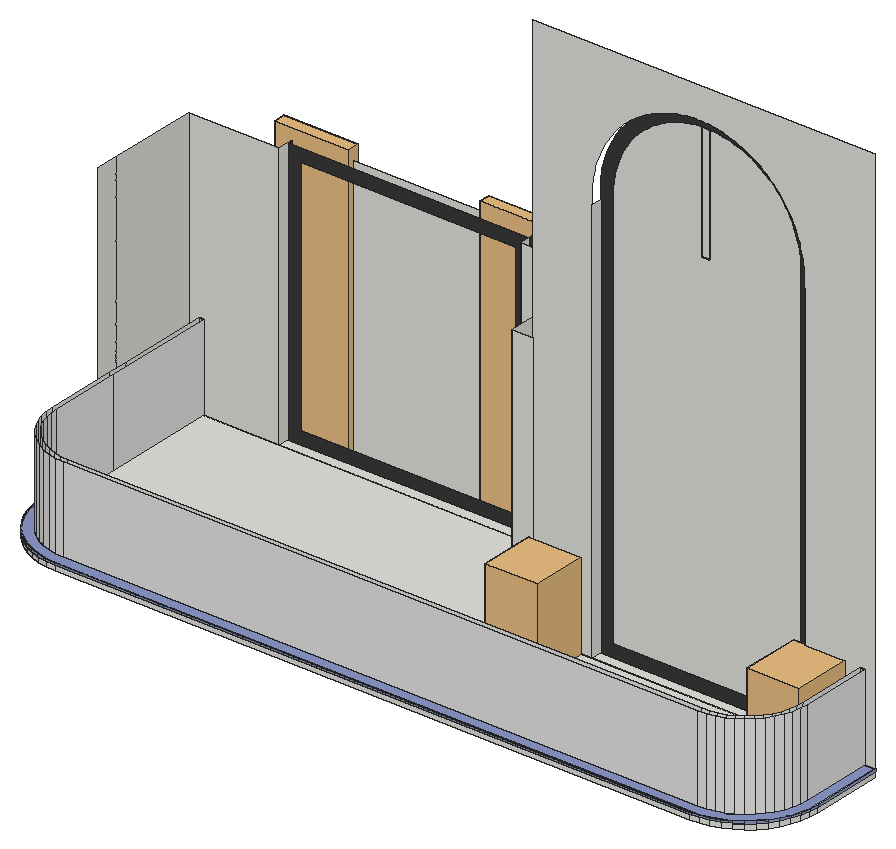
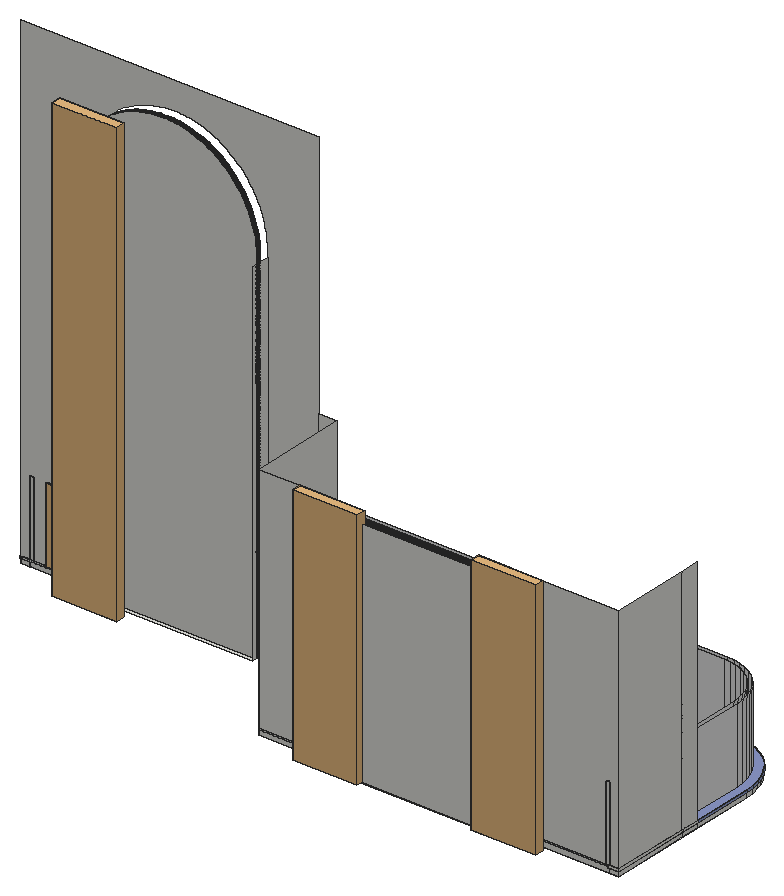
# SketchUp Ruby script. Lengths in inches.
U = 1.inch
M = Sketchup.active_model
def pt(a) = Geom::Point3d.new(a.map { |v| v * U })
def face(e, loops, mat)
  f = e.add_face(loops[0].map { |a| pt(a) })
  loops[1..].each { |l| e.add_face(l.map { |a| pt(a) }).erase! }
  f.material = f.back_material = mat if mat
  f
end
# faces: each face lists its corners as indices into pts; further lists are holes
def faces(e, pts, list, mat = nil) = list.each { |f| face(e, (f[0].is_a?(Array) ? f : [f]).map { |l| l.map { |i| pts[i] } }, mat) }
# xy, xz, yz: faces in a plane at the given z, y or x. An outline is a flat list of corners, or four numbers for a rectangle; further outlines are holes
def ring(l) = l.size == 4 ? [[l[0], l[1]], [l[2], l[1]], [l[2], l[3]], [l[0], l[3]]] : l.each_slice(2).to_a
def flat(e, list, mat, &to3) = list.each { |f| face(e, (f[0].is_a?(Array) ? f : [f]).map { |l| ring(l).map { |u, v| to3.(u, v) } }, mat) }
def xy(e, z, list, mat = nil) = flat(e, list, mat) { |x, y| [x, y, z] }
def xz(e, y, list, mat = nil) = flat(e, list, mat) { |x, z| [x, y, z] }
def yz(e, x, list, mat = nil) = flat(e, list, mat) { |y, z| [x, y, z] }
def lines(e, pts, list) = list.each { |a, b| e.add_line(pt(pts[a]), pt(pts[b])) }
# prism: a flat outline (further loops are holes) pulled along v
def prism(e, loops, v, mat = nil)
  f = face(e, loops, mat); d = Geom::Vector3d.new(v.map { |x| x * U })
  f.pushpull(f.normal.samedirection?(d) ? d.length : -d.length)
end
def box(e, o, s, mat = nil) = prism(e, [[o, [o[0] + s[0], o[1], o[2]], [o[0] + s[0], o[1] + s[1], o[2]], [o[0], o[1] + s[1], o[2]]]], [0, 0, s[2]], mat)
def at(x, y, z, deg = 0) = Geom::Transformation.translation(pt([x, y, z])) * Geom::Transformation.rotation(ORIGIN, Z_AXIS, deg.degrees)
def axes(o, x, y, z) = Geom::Transformation.new([*x, 0, *y, 0, *z, 0, *pt(o).to_a, 1])
def part(name) = M.definitions.add(name)
# library, detail: a bought-in or finely detailed component or shape, given as its bounding box
def library(name, o, s) = part(name).tap { |d| box(d.entities, o, s) }
def detail(e, o, s) = box(e.add_group.entities, o, s)
def put(e, d, t, mat = nil) = e.add_instance(d, t).tap { |i| i.material = mat if mat }
def group(e, t, mat = nil) = e.add_group.tap { |g| g.transformation = t; g.material = mat if mat }.entities
root = M.entities
M.materials.add("0326 AP 7207 CLASSIC PURPLE").color = [140, 152, 201]
M.materials.add("[Color M07]").color = [58, 58, 58]
M.materials.add("[Mirror 02]").color = [229, 229, 229]
c1 = library("Curtains 004",[-15.59,-2.26,0],[31.18,4.52,116.91])
c2 = library("Ficus elastica Belize 002",[-7.92,-8.8125,0.01],[22.14,24.73,36.43])
xy(root,136.75,[[220.41,26.25,487.41,26.25,491.32,26.51,495.17,27.27,498.89,28.53,502.41,30.27,505.67,32.45,508.62,35.04,511.21,37.99,513.39,41.25,515.125,44.77,516.38,48.49,517.15,52.33,517.41,56.25,517.41,86.25,364.41,86.25,364.41,133.75,190.41,133.75,190.41,56.25,190.66,52.33,191.43,48.49,192.69,44.77,194.43,41.25,196.61,37.99,199.19,35.04,202.14,32.45,205.41,30.27,208.93,28.53,212.64,27.27,216.49,26.51]])
xy(root,139.125,[[220.41,25.95,487.41,25.95,491.36,26.21,495.25,26.98,499,28.25,502.56,30.01,505.85,32.21,508.83,34.82,511.45,37.8,513.65,41.1,515.4,44.65,516.68,48.41,517.45,52.29,517.71,56.25,517.71,86.55,512.71,86.55,512.71,86.25,517.41,86.25,517.41,56.25,517.15,52.33,516.38,48.49,515.125,44.77,513.39,41.25,511.21,37.99,508.62,35.04,505.67,32.45,502.41,30.27,498.89,28.53,495.17,27.27,491.32,26.51,487.41,26.25,220.41,26.25,216.49,26.51,212.64,27.27,208.93,28.53,205.41,30.27,202.14,32.45,199.19,35.04,196.61,37.99,194.43,41.25,192.69,44.77,191.43,48.49,190.66,52.33,190.41,56.25,190.41,133.75,195.11,133.75,195.11,134.05,190.1,134.05,190.1,56.25,190.36,52.29,191.14,48.41,192.41,44.65,194.16,41.1,196.37,37.8,198.98,34.82,201.96,32.21,205.26,30.01,208.81,28.25,212.5625,26.98,216.45,26.21],[220.41,26.25,487.41,26.25,491.32,26.51,495.17,27.27,498.89,28.53,502.41,30.27,505.67,32.45,508.62,35.04,511.21,37.99,513.39,41.25,515.125,44.77,516.38,48.49,517.15,52.33,517.41,56.25,517.41,86.25,364.41,86.25,364.41,133.75,190.41,133.75,190.41,56.25,190.66,52.33,191.43,48.49,192.69,44.77,194.43,41.25,196.61,37.99,199.19,35.04,202.14,32.45,205.41,30.27,208.93,28.53,212.64,27.27,216.49,26.51]])
xy(root,140.0625,[[220.41,30.65,217.06,30.87,213.78,31.52,210.61,32.6,207.6,34.08,204.82,35.9375,202.3,38.15,200.09,40.66,198.23,43.45,196.75,46.45,195.68,49.625,195.02,52.91,194.8,56.25,194.8,133.75,195.11,133.75,195.11,56.25,195.32,52.95,195.97,49.7,197.03,46.57,198.5,43.6,200.33,40.85,202.52,38.36,205,36.18,207.76,34.34,210.72,32.875,213.86,31.8125,217.1,31.17,220.41,30.95,487.41,30.95,490.71,31.17,493.96,31.8125,497.09,32.875,500.06,34.34,502.81,36.18,505.3,38.36,507.48,40.85,509.32,43.6,510.78,46.57,511.85,49.7,512.49,52.95,512.71,56.25,512.71,86.25,513.01,86.25,513.01,56.25,512.79,52.91,512.14,49.625,511.0625,46.45,509.58,43.45,507.72,40.66,505.51,38.15,502.99,35.9375,500.21,34.08,497.2,32.6,494.03,31.52,490.75,30.87,487.41,30.65],[220.41,30.95,217.1,31.17,213.86,31.8125,210.72,32.875,207.76,34.34,205,36.18,202.52,38.36,200.33,40.85,198.5,43.6,197.03,46.57,195.97,49.7,195.32,52.95,195.11,56.25,195.11,133.75,196.73,133.75,196.73,56.25,196.9375,53.16,197.54,50.12,198.54,47.19,199.9,44.41,201.625,41.84,203.67,39.51,206,37.47,208.57,35.75,211.35,34.38,214.28,33.38,217.32,32.78,220.41,32.58,487.41,32.58,490.5,32.78,493.53,33.38,496.47,34.38,499.24,35.75,501.82,37.47,504.15,39.51,506.1875,41.84,507.91,44.41,509.28,47.19,510.27,50.12,510.88,53.16,511.08,56.25,511.08,86.25,512.71,86.25,512.71,56.25,512.49,52.95,511.85,49.7,510.78,46.57,509.32,43.6,507.48,40.85,505.3,38.36,502.81,36.18,500.06,34.34,497.09,32.875,493.96,31.8125,490.71,31.17,487.41,30.95],[220.41,32.58,487.41,32.58,490.5,32.78,493.53,33.38,496.47,34.38,499.24,35.75,501.82,37.47,504.15,39.51,506.1875,41.84,507.91,44.41,509.28,47.19,510.27,50.12,510.88,53.16,511.08,56.25,511.08,86.25,364.41,86.25,364.41,133.75,196.73,133.75,196.73,56.25,196.9375,53.16,197.54,50.12,198.54,47.19,199.9,44.41,201.625,41.84,203.67,39.51,206,37.47,208.57,35.75,211.35,34.38,214.28,33.38,217.32,32.78],[398.23,86.25,487.79,90.75],[398.23,90.75,487.79,93.1875],
  [398.23,93.1875,487.79,95.25],[228.58,133.75,330.09,138.25],[228.58,138.25,330.09,142.3125],[228.58,142.3125,330.09,142.75]])
xy(root,140.0625,[[220.41,25.95,487.41,25.95,491.36,26.21,495.25,26.98,499,28.25,502.56,30.01,505.85,32.21,508.83,34.82,511.45,37.8,513.65,41.1,515.4,44.65,516.68,48.41,517.45,52.29,517.71,56.25,517.71,86.55,512.71,86.55,512.71,86.25,517.41,86.25,517.41,56.25,517.15,52.33,516.38,48.49,515.125,44.77,513.39,41.25,511.21,37.99,508.62,35.04,505.67,32.45,502.41,30.27,498.89,28.53,495.17,27.27,491.32,26.51,487.41,26.25,220.41,26.25,216.49,26.51,212.64,27.27,208.93,28.53,205.41,30.27,202.14,32.45,199.19,35.04,196.61,37.99,194.43,41.25,192.69,44.77,191.43,48.49,190.66,52.33,190.41,56.25,190.41,133.75,195.11,133.75,195.11,134.05,190.1,134.05,190.1,56.25,190.36,52.29,191.14,48.41,192.41,44.65,194.16,41.1,196.37,37.8,198.98,34.82,201.96,32.21,205.26,30.01,208.81,28.25,212.5625,26.98,216.45,26.21],[220.41,26.25,487.41,26.25,491.32,26.51,495.17,27.27,498.89,28.53,502.41,30.27,505.67,32.45,508.62,35.04,511.21,37.99,513.39,41.25,515.125,44.77,516.38,48.49,517.15,52.33,517.41,56.25,517.41,86.25,513.01,86.25,513.01,56.25,512.79,52.91,512.14,49.625,511.0625,46.45,509.58,43.45,507.72,40.66,505.51,38.15,502.99,35.9375,500.21,34.08,497.2,32.6,494.03,31.52,490.75,30.87,487.41,30.65,220.41,30.65,217.06,30.87,213.78,31.52,210.61,32.6,207.6,34.08,204.82,35.9375,202.3,38.15,200.09,40.66,198.23,43.45,196.75,46.45,195.68,49.625,195.02,52.91,194.8,56.25,194.8,133.75,190.41,133.75,190.41,56.25,190.66,52.33,191.43,48.49,192.69,44.77,194.43,41.25,196.61,37.99,199.19,35.04,202.14,32.45,205.41,30.27,208.93,28.53,212.64,27.27,216.49,26.51]],"0326 AP 7207 CLASSIC PURPLE")
xz(root,25.95,[[220.41,139.125,487.41,140.0625]],"0326 AP 7207 CLASSIC PURPLE")
xz(root,26.25,[[220.41,136.75,487.41,139.125],[220.41,139.125,487.41,140.0625]])
xz(root,30.65,[[220.41,140.0625,487.41,176.0625]],"[Mirror 02]")
xz(root,32.58,[[220.41,140.0625,487.41,176.0625]],"[Mirror 02]")
xz(root,86.25,[[364.41,136.75,373.41,139.125],[373.41,136.75,398.23,139.125],[398.23,136.75,487.79,139.125],[487.79,136.75,512.71,139.125],[512.71,136.75,513.01,139.125],
  [513.01,136.75,517.41,139.125],[364.41,139.125,373.41,140.0625],[373.41,139.125,398.23,140.0625],[398.23,139.125,487.79,140.0625],[487.79,139.125,512.71,140.0625],
  [512.71,139.125,513.01,140.0625],[513.01,139.125,517.41,140.0625],[364.41,140.0625,373.41,252],[373.41,140.0625,398.23,140.0625,398.23,311,398.15,312.47,398.13,313.94,398.15,315.41,398.22,316.88,398.23,316.97,398.23,311,398.15,312.47,398.13,313.94,398.15,315.41,398.22,316.88,398.23,316.97,398.34,318.34,398.51,319.8,398.72,321.26,398.98,322.7,399.29,324.14,399.65,325.57,400.05,326.98,400.5,328.38,400.99,329.77,401.53,331.13,402.11,332.48,402.74,333.8125,403.41,335.12,404.125,336.41,404.88,337.67,405.67,338.9,406.51,340.11,407.38,341.29,408.3,342.44,409.25,343.57,410.23,344.66,411.25,345.71,412.31,346.74,413.4,347.72,414.52,348.67,415.67,349.59,416.85,350.47,418.06,351.3,419.29,352.1,420.55,352.86,421.84,353.57,423.14,354.24,424.47,354.87,425.82,355.46,427.1875,356,428.57,356.49,429.97,356.94,431.38,357.35,432.8125,357.7,434.25,358.01,435.69,358.28,437.15,358.49,438.61,358.66,440.07,358.78,441.54,358.85,443.01,358.88,444.48,358.85,445.95,358.78,447.41,358.66,448.87,358.49,450.33,358.28,451.77,358.01,453.21,357.7,454.64,357.35,456.05,356.94,457.45,356.49,458.83,356,460.2,355.46,461.55,354.87,462.875,354.24,464.18,353.57,465.47,352.86,466.73,352.1,467.96,351.3,469.17,350.47,470.35,349.59,471.5,348.67,472.62,347.72,473.71,346.74,474.77,345.71,475.79,344.66,476.77,343.57,477.72,342.44,478.64,341.29,479.51,340.11,480.35,338.9,481.14,337.67,481.9,336.41,482.61,335.12,483.28,333.8125,483.91,332.48,484.49,331.13,485.03,329.77,485.52,328.38,485.97,326.98,486.375,325.57,486.73,324.14,487.04,322.7,487.3,321.26,487.51,319.8,487.68,318.34,487.79,316.97,487.8,316.88,487.87,315.41,487.89,313.94,487.87,312.47,487.79,311,487.79,316.97,487.8,316.88,487.87,315.41,487.89,313.94,487.87,312.47,487.79,311,487.79,140.0625,511.08,140.0625,511.08,176.5,513.01,176.5,513.01,140.0625,517.41,140.0625,517.41,372,373.41,372],[511.08,140.0625,513.01,176.0625]])
xz(root,86.55,[[512.71,139.125,517.71,140.0625]])
xz(root,90.75,[[[398.23,140.0625,487.79,140.0625,487.79,316.97,487.68,318.34,487.51,319.8,487.3,321.26,487.04,322.7,486.73,324.14,486.375,325.57,485.97,326.98,485.52,328.38,485.03,329.77,484.49,331.13,483.91,332.48,483.28,333.8125,482.61,335.12,481.9,336.41,481.14,337.67,480.35,338.9,479.51,340.11,478.64,341.29,477.72,342.44,476.77,343.57,475.79,344.66,474.77,345.71,473.71,346.74,472.62,347.72,471.5,348.67,470.35,349.59,469.17,350.47,467.96,351.3,466.73,352.1,465.47,352.86,464.18,353.57,462.875,354.24,461.55,354.87,460.2,355.46,458.83,356,457.45,356.49,456.05,356.94,454.64,357.35,453.21,357.7,451.77,358.01,450.33,358.28,448.87,358.49,447.41,358.66,445.95,358.78,444.48,358.85,443.01,358.88,441.54,358.85,440.07,358.78,438.61,358.66,437.15,358.49,435.69,358.28,434.25,358.01,432.8125,357.7,431.38,357.35,429.97,356.94,428.57,356.49,427.1875,356,425.82,355.46,424.47,354.87,423.14,354.24,421.84,353.57,420.55,352.86,419.29,352.1,418.06,351.3,416.85,350.47,415.67,349.59,414.52,348.67,413.4,347.72,412.31,346.74,411.25,345.71,410.23,344.66,409.25,343.57,408.3,342.44,407.38,341.29,406.51,340.11,405.67,338.9,404.88,337.67,404.125,336.41,403.41,335.12,402.74,333.8125,402.11,332.48,401.53,331.13,400.99,329.77,400.5,328.38,400.05,326.98,399.65,325.57,399.29,324.14,398.98,322.7,398.72,321.26,398.51,319.8,398.34,318.34,398.23,316.97],[403.41,145.24,403.41,316.76,403.5,317.84,403.64,319.13,403.83,320.42,404.0625,321.7,404.34,322.97,404.65,324.23,405.01,325.48,405.4,326.72,405.84,327.95,406.32,329.16,406.83,330.35,407.39,331.52,407.98,332.68,408.61,333.82,409.28,334.93,409.98,336.03,410.72,337.1,411.5,338.14,412.3,339.16,413.14,340.15,414.02,341.12,414.92,342.05,415.85,342.96,416.82,343.83,417.81,344.67,418.82,345.48,419.87,346.26,420.9375,347,422.03,347.7,423.14,348.37,424.28,349,425.4375,349.6,426.61,350.15,427.81,350.67,429.01,351.15,430.24,351.59,431.48,351.99,432.73,352.34,433.99,352.66,435.26,352.93,436.54,353.17,437.82,353.36,439.12,353.51,440.41,353.61,441.71,353.68,443.01,353.7,444.31,353.68,445.61,353.61,446.9,353.51,448.2,353.36,449.48,353.17,450.76,352.93,452.03,352.66,453.29,352.34,454.54,351.99,455.78,351.59,457.01,351.15,458.21,350.67,459.41,350.15,460.58,349.6,461.74,349,462.875,348.37,463.99,347.7,465.08,347,466.15,346.26,467.2,345.48,468.21,344.67,469.2,343.83,470.17,342.96,471.1,342.05,472,341.12,472.875,340.15,473.72,339.16,474.53,338.14,475.3,337.1,476.04,336.03,476.74,334.93,477.41,333.82,478.04,332.68,478.63,331.52,479.1875,330.35,479.7,329.16,480.18,327.95,480.62,326.72,481.01,325.48,481.37,324.23,481.68,322.97,481.96,321.7,482.1875,320.42,482.38,319.13,482.52,317.84,482.61,316.76,482.61,145.24],[440.73,304.37,440.73,353.61,444.31,353.68,444.31,304.37]]],"[Color M07]")
xz(root,93.1875,[[398.23,140.0625,398.23,316.97,398.34,318.34,398.51,319.8,398.72,321.26,398.98,322.7,399.29,324.14,399.65,325.57,400.05,326.98,400.5,328.38,400.99,329.77,401.53,331.13,402.11,332.48,402.74,333.8125,403.41,335.12,404.125,336.41,404.88,337.67,405.67,338.9,406.51,340.11,407.38,341.29,408.3,342.44,409.25,343.57,410.23,344.66,411.25,345.71,412.31,346.74,413.4,347.72,414.52,348.67,415.67,349.59,416.85,350.47,418.06,351.3,419.29,352.1,420.55,352.86,421.84,353.57,423.14,354.24,424.47,354.87,425.82,355.46,427.1875,356,428.57,356.49,429.97,356.94,431.38,357.35,432.8125,357.7,434.25,358.01,435.69,358.28,437.15,358.49,438.61,358.66,440.07,358.78,441.54,358.85,443.01,358.88,444.48,358.85,445.95,358.78,447.41,358.66,448.87,358.49,450.33,358.28,451.77,358.01,453.21,357.7,454.64,357.35,456.05,356.94,457.45,356.49,458.83,356,460.2,355.46,461.55,354.87,462.875,354.24,464.18,353.57,465.47,352.86,466.73,352.1,467.96,351.3,469.17,350.47,470.35,349.59,471.5,348.67,472.62,347.72,473.71,346.74,474.77,345.71,475.79,344.66,476.77,343.57,477.72,342.44,478.64,341.29,479.51,340.11,480.35,338.9,481.14,337.67,481.9,336.41,482.61,335.12,483.28,333.8125,483.91,332.48,484.49,331.13,485.03,329.77,485.52,328.38,485.97,326.98,486.375,325.57,486.73,324.14,487.04,322.7,487.3,321.26,487.51,319.8,487.68,318.34,487.79,316.97,487.79,140.0625]])
xz(root,133.75,[[190.41,136.75,194.8,139.125],[194.8,136.75,195.11,139.125],[195.11,136.75,364.41,139.125],[190.41,139.125,194.8,140.0625],[194.8,139.125,195.11,140.0625],
  [195.11,139.125,364.41,140.0625],[190.41,140.0625,194.8,140.0625,194.8,176.5,196.73,176.5,196.73,140.0625,228.58,140.0625,228.58,252,190.41,252],[194.8,140.0625,196.73,176.0625],[330.09,140.0625,364.41,252]])
xz(root,134.05,[[190.1,139.125,195.11,140.0625]])
xz(root,138.25,[[[228.58,140.0625,330.09,252],[233.89,145.37,324.79,246.69]]],"[Color M07]")
xz(root,142.3125,[[228.58,140.0625,330.09,252]])
yz(root,190.1,[[86.25,139.125,95.25,140.0625],[95.25,139.125,134.05,140.0625]])
yz(root,190.1,[[56.25,139.125,86.25,140.0625]],"0326 AP 7207 CLASSIC PURPLE")
yz(root,190.41,[[56.25,136.75,86.25,139.125],[86.25,136.75,95.25,139.125],[95.25,136.75,133.75,139.125],[56.25,139.125,86.25,140.0625],[86.25,139.125,95.25,140.0625],
  [95.25,139.125,133.75,140.0625],[86.25,140.0625,95.25,252],[95.25,140.0625,133.75,252]])
yz(root,194.8,[[95.25,140.0625,133.75,176.0625]])
yz(root,194.8,[[56.25,140.0625,86.25,176.0625],[86.25,140.0625,95.25,176.0625]],"[Mirror 02]")
yz(root,195.11,[[133.75,139.125,134.05,140.0625]])
yz(root,196.73,[[56.25,140.0625,86.25,176.0625],[86.25,140.0625,133.75,176.0625]],"[Mirror 02]")
yz(root,228.58,[[133.75,140.0625,138.25,252],[142.3125,140.0625,142.75,252]])
yz(root,228.58,[[138.25,140.0625,142.3125,252]],"[Color M07]")
yz(root,330.09,[[133.75,140.0625,138.25,252],[142.3125,140.0625,142.75,252]])
yz(root,330.09,[[138.25,140.0625,142.3125,252]],"[Color M07]")
yz(root,364.41,[[86.25,136.75,133.75,139.125],[86.25,139.125,133.75,140.0625],[86.25,140.0625,133.75,252]])
yz(root,398.23,[[86.25,140.0625,90.75,311],[93.1875,140.0625,95.25,311]])
yz(root,398.23,[[90.75,140.0625,93.1875,311]],"[Color M07]")
yz(root,487.79,[[86.25,140.0625,90.75,311],[93.1875,140.0625,95.25,311]])
yz(root,487.79,[[90.75,140.0625,93.1875,311]],"[Color M07]")
yz(root,511.08,[[56.25,140.0625,86.25,176.0625]],"[Mirror 02]")
yz(root,512.71,[[86.25,139.125,86.55,140.0625]])
yz(root,513.01,[[56.25,140.0625,86.25,176.0625]],"[Mirror 02]")
yz(root,517.41,[[56.25,136.75,86.25,139.125],[56.25,139.125,86.25,140.0625]])
yz(root,517.71,[[56.25,139.125,86.55,140.0625]],"0326 AP 7207 CLASSIC PURPLE")
p = [[220.41,26.25,139.125],[220.41,26.25,136.75],[216.49,26.51,136.75],[216.49,26.51,139.125],[491.32,26.51,139.125],[491.32,26.51,136.75],
  [487.41,26.25,136.75],[487.41,26.25,139.125],[212.64,27.27,136.75],[212.64,27.27,139.125],[495.17,27.27,139.125],[495.17,27.27,136.75],
  [208.93,28.53,136.75],[208.93,28.53,139.125],[498.89,28.53,139.125],[498.89,28.53,136.75],[205.41,30.27,136.75],[205.41,30.27,139.125],
  [502.41,30.27,139.125],[502.41,30.27,136.75],[202.14,32.45,136.75],[202.14,32.45,139.125],[505.67,32.45,139.125],[505.67,32.45,136.75],
  [199.19,35.04,136.75],[199.19,35.04,139.125],[508.62,35.04,139.125],[508.62,35.04,136.75],[196.61,37.99,136.75],[196.61,37.99,139.125],
  [511.21,37.99,139.125],[511.21,37.99,136.75],[194.43,41.25,136.75],[194.43,41.25,139.125],[513.39,41.25,139.125],[513.39,41.25,136.75],
  [192.69,44.77,136.75],[192.69,44.77,139.125],[515.125,44.77,139.125],[515.125,44.77,136.75],[191.43,48.49,136.75],[191.43,48.49,139.125],
  [516.38,48.49,139.125],[516.38,48.49,136.75],[190.66,52.33,136.75],[190.66,52.33,139.125],[517.15,52.33,139.125],[517.15,52.33,136.75],
  [190.41,56.25,136.75],[190.41,56.25,139.125],[517.41,56.25,139.125],[517.41,56.25,136.75],[220.41,25.95,140.0625],[216.45,26.21,140.0625],
  [216.45,26.21,139.125],[220.41,25.95,139.125],[491.36,26.21,140.0625],[487.41,25.95,140.0625],[487.41,25.95,139.125],[491.36,26.21,139.125],
  [212.5625,26.98,140.0625],[212.5625,26.98,139.125],[216.49,26.51,140.0625],[220.41,26.25,140.0625],[487.41,26.25,140.0625],[491.32,26.51,140.0625],
  [495.25,26.98,140.0625],[495.25,26.98,139.125],[212.64,27.27,140.0625],[495.17,27.27,140.0625],[208.81,28.25,140.0625],[208.81,28.25,139.125],
  [499,28.25,140.0625],[499,28.25,139.125],[208.93,28.53,140.0625],[498.89,28.53,140.0625],[205.26,30.01,140.0625],[205.26,30.01,139.125],
  [502.56,30.01,140.0625],[502.56,30.01,139.125],[205.41,30.27,140.0625],[502.41,30.27,140.0625],[201.96,32.21,140.0625],[201.96,32.21,139.125],
  [505.85,32.21,140.0625],[505.85,32.21,139.125],[202.14,32.45,140.0625],[505.67,32.45,140.0625],[198.98,34.82,140.0625],[198.98,34.82,139.125],
  [508.83,34.82,140.0625],[508.83,34.82,139.125],[199.19,35.04,140.0625],[508.62,35.04,140.0625],[196.37,37.8,140.0625],[196.37,37.8,139.125],
  [511.45,37.8,140.0625],[511.45,37.8,139.125],[196.61,37.99,140.0625],[511.21,37.99,140.0625],[194.16,41.1,140.0625],[194.16,41.1,139.125],
  [513.65,41.1,140.0625],[513.65,41.1,139.125],[194.43,41.25,140.0625],[513.39,41.25,140.0625],[192.41,44.65,140.0625],[192.41,44.65,139.125],
  [515.4,44.65,140.0625],[515.4,44.65,139.125],[192.69,44.77,140.0625],[515.125,44.77,140.0625],[191.14,48.41,140.0625],[191.14,48.41,139.125],
  [516.68,48.41,140.0625],[516.68,48.41,139.125],[191.43,48.49,140.0625],[516.38,48.49,140.0625],[190.36,52.29,140.0625],[190.36,52.29,139.125],
  [517.45,52.29,140.0625],[517.45,52.29,139.125],[190.66,52.33,140.0625],[517.15,52.33,140.0625],[190.1,56.25,140.0625],[190.1,56.25,139.125],
  [190.41,56.25,140.0625],[517.41,56.25,140.0625],[517.71,56.25,140.0625],[517.71,56.25,139.125],[217.06,30.87,140.0625],[220.41,30.65,140.0625],
  [220.41,30.65,176.0625],[217.06,30.87,176.0625],[487.41,30.65,140.0625],[490.75,30.87,140.0625],[490.75,30.87,176.0625],[487.41,30.65,176.0625],
  [213.78,31.52,140.0625],[213.78,31.52,176.0625],[494.03,31.52,140.0625],[494.03,31.52,176.0625],[210.61,32.6,140.0625],[210.61,32.6,176.0625],
  [497.2,32.6,140.0625],[497.2,32.6,176.0625],[207.6,34.08,140.0625],[207.6,34.08,176.0625],[220.41,32.58,140.0625],[217.32,32.78,140.0625],
  [217.32,32.78,176.0625],[220.41,32.58,176.0625],[490.5,32.78,140.0625],[487.41,32.58,140.0625],[487.41,32.58,176.0625],[490.5,32.78,176.0625],
  [500.21,34.08,140.0625],[500.21,34.08,176.0625],[214.28,33.38,140.0625],[214.28,33.38,176.0625],[493.53,33.38,140.0625],[493.53,33.38,176.0625],
  [211.35,34.38,140.0625],[211.35,34.38,176.0625],[496.47,34.38,140.0625],[496.47,34.38,176.0625],[204.82,35.9375,140.0625],[204.82,35.9375,176.0625],
  [502.99,35.9375,140.0625],[502.99,35.9375,176.0625],[208.57,35.75,140.0625],[208.57,35.75,176.0625],[499.24,35.75,140.0625],[499.24,35.75,176.0625],
  [206,37.47,140.0625],[206,37.47,176.0625],[501.82,37.47,140.0625],[501.82,37.47,176.0625],[202.3,38.15,140.0625],[202.3,38.15,176.0625],
  [505.51,38.15,140.0625],[505.51,38.15,176.0625],[203.67,39.51,140.0625],[203.67,39.51,176.0625],[504.15,39.51,140.0625],[504.15,39.51,176.0625],
  [200.09,40.66,140.0625],[200.09,40.66,176.0625],[507.72,40.66,140.0625],[507.72,40.66,176.0625],[201.625,41.84,140.0625],[201.625,41.84,176.0625],
  [506.1875,41.84,140.0625],[506.1875,41.84,176.0625],[198.23,43.45,140.0625],[198.23,43.45,176.0625],[509.58,43.45,140.0625],[509.58,43.45,176.0625],
  [199.9,44.41,140.0625],[199.9,44.41,176.0625],[507.91,44.41,140.0625],[507.91,44.41,176.0625],[196.75,46.45,140.0625],[196.75,46.45,176.0625],
  [511.0625,46.45,140.0625],[511.0625,46.45,176.0625],[198.54,47.19,140.0625],[198.54,47.19,176.0625],[509.28,47.19,140.0625],[509.28,47.19,176.0625],
  [195.68,49.625,140.0625],[195.68,49.625,176.0625],[512.14,49.625,140.0625],[512.14,49.625,176.0625],[197.54,50.12,140.0625],[197.54,50.12,176.0625],
  [510.27,50.12,140.0625],[510.27,50.12,176.0625],[195.02,52.91,140.0625],[195.02,52.91,176.0625],[512.79,52.91,140.0625],[512.79,52.91,176.0625],
  [196.9375,53.16,140.0625],[196.9375,53.16,176.0625],[510.88,53.16,140.0625],[510.88,53.16,176.0625],[194.8,56.25,140.0625],[194.8,56.25,176.0625],
  [513.01,56.25,140.0625],[513.01,56.25,176.0625],[196.73,56.25,140.0625],[196.73,56.25,176.0625],[511.08,56.25,140.0625],[511.08,56.25,176.0625]]
faces(root,p,[[0,1,2,3],[4,5,6,7],[3,2,8,9],[10,11,5,4],[9,8,12,13],[14,15,11,10],[13,12,16,17],[18,19,15,14],
  [17,16,20,21],[22,23,19,18],[21,20,24,25],[26,27,23,22],[25,24,28,29],[30,31,27,26],[29,28,32,33],[34,35,31,30],
  [33,32,36,37],[38,39,35,34],[37,36,40,41],[42,43,39,38],[41,40,44,45],[46,47,43,42],[45,44,48,49],[50,51,47,46],
  [62,3,0,63],[64,7,4,65],[68,9,3,62],[65,4,10,69],[74,13,9,68],[69,10,14,75],[80,17,13,74],[75,14,18,81],
  [86,21,17,80],[81,18,22,87],[92,25,21,86],[87,22,26,93],[98,29,25,92],[93,26,30,99],[104,33,29,98],[99,30,34,105],
  [110,37,33,104],[105,34,38,111],[116,41,37,110],[111,38,42,117],[122,45,41,116],[117,42,46,123],[126,49,45,122],[123,46,50,127]])
faces(root,p,[[52,53,54,55],[56,57,58,59],[53,60,61,54],[66,56,59,67],[60,70,71,61],[72,66,67,73],[70,76,77,71],[78,72,73,79],
  [76,82,83,77],[84,78,79,85],[82,88,89,83],[90,84,85,91],[88,94,95,89],[96,90,91,97],[94,100,101,95],[102,96,97,103],
  [100,106,107,101],[108,102,103,109],[106,112,113,107],[114,108,109,115],[112,118,119,113],[120,114,115,121],[118,124,125,119],[128,120,121,129]],"0326 AP 7207 CLASSIC PURPLE")
faces(root,p,[[130,131,132,133],[134,135,136,137],[138,130,133,139],[135,140,141,136],[142,138,139,143],[140,144,145,141],[146,142,143,147],[148,149,150,151],
  [152,153,154,155],[144,156,157,145],[149,158,159,150],[160,152,155,161],[158,162,163,159],[164,160,161,165],[166,146,147,167],[156,168,169,157],
  [162,170,171,163],[172,164,165,173],[170,174,175,171],[176,172,173,177],[178,166,167,179],[168,180,181,169],[174,182,183,175],[184,176,177,185],
  [186,178,179,187],[180,188,189,181],[182,190,191,183],[192,184,185,193],[194,186,187,195],[188,196,197,189],[190,198,199,191],[200,192,193,201],
  [202,194,195,203],[196,204,205,197],[198,206,207,199],[208,200,201,209],[210,202,203,211],[204,212,213,205],[206,214,215,207],[216,208,209,217],
  [218,210,211,219],[212,220,221,213],[214,222,223,215],[224,216,217,225],[226,218,219,227],[220,228,229,221],[222,230,231,223],[232,224,225,233]],"[Mirror 02]")
put(root,c1,axes([476.69,96.5,136.8125],[1,0,0],[0,1,0],[0,0,1.83]))
put(root,c1,at(323.41,142.75,140.0625))
put(root,c1,at(237.05,142.75,140.0625))
put(root,c2,at(490.5,70.92,140.0625))
put(root,c2,at(379.45,72.07,140.0625))
